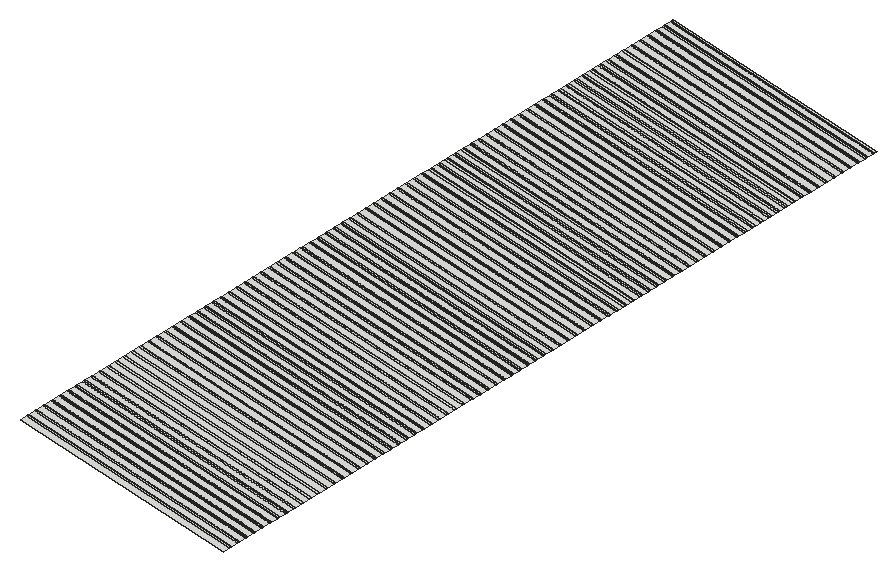
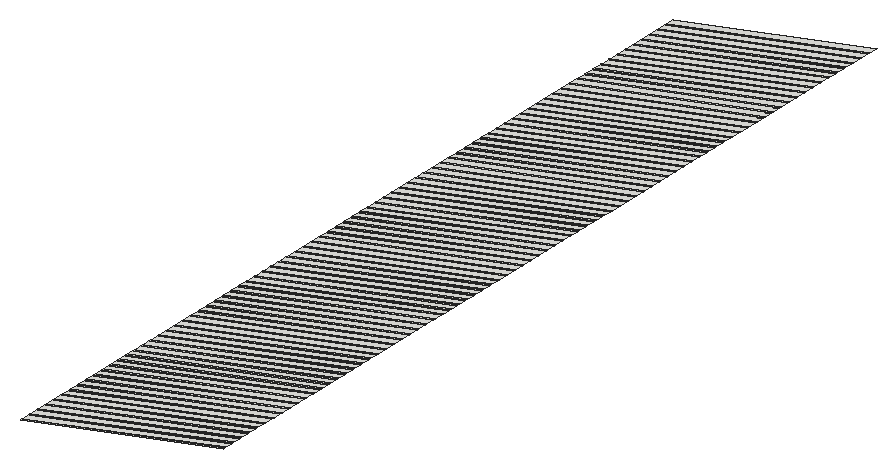
# SketchUp Ruby script. Lengths in inches.
U = 1.inch
M = Sketchup.active_model
def pt(a) = Geom::Point3d.new(a.map { |v| v * U })
def face(e, loops, mat)
  f = e.add_face(loops[0].map { |a| pt(a) })
  loops[1..].each { |l| e.add_face(l.map { |a| pt(a) }).erase! }
  f.material = f.back_material = mat if mat
  f
end
# faces: each face lists its corners as indices into pts; further lists are holes
def faces(e, pts, list, mat = nil) = list.each { |f| face(e, (f[0].is_a?(Array) ? f : [f]).map { |l| l.map { |i| pts[i] } }, mat) }
# xy, xz, yz: faces in a plane at the given z, y or x. An outline is a flat list of corners, or four numbers for a rectangle; further outlines are holes
def ring(l) = l.size == 4 ? [[l[0], l[1]], [l[2], l[1]], [l[2], l[3]], [l[0], l[3]]] : l.each_slice(2).to_a
def flat(e, list, mat, &to3) = list.each { |f| face(e, (f[0].is_a?(Array) ? f : [f]).map { |l| ring(l).map { |u, v| to3.(u, v) } }, mat) }
def xy(e, z, list, mat = nil) = flat(e, list, mat) { |x, y| [x, y, z] }
def xz(e, y, list, mat = nil) = flat(e, list, mat) { |x, z| [x, y, z] }
def yz(e, x, list, mat = nil) = flat(e, list, mat) { |y, z| [x, y, z] }
def lines(e, pts, list) = list.each { |a, b| e.add_line(pt(pts[a]), pt(pts[b])) }
# prism: a flat outline (further loops are holes) pulled along v
def prism(e, loops, v, mat = nil)
  f = face(e, loops, mat); d = Geom::Vector3d.new(v.map { |x| x * U })
  f.pushpull(f.normal.samedirection?(d) ? d.length : -d.length)
end
def box(e, o, s, mat = nil) = prism(e, [[o, [o[0] + s[0], o[1], o[2]], [o[0] + s[0], o[1] + s[1], o[2]], [o[0], o[1] + s[1], o[2]]]], [0, 0, s[2]], mat)
def at(x, y, z, deg = 0) = Geom::Transformation.translation(pt([x, y, z])) * Geom::Transformation.rotation(ORIGIN, Z_AXIS, deg.degrees)
def axes(o, x, y, z) = Geom::Transformation.new([*x, 0, *y, 0, *z, 0, *pt(o).to_a, 1])
def part(name) = M.definitions.add(name)
# library, detail: a bought-in or finely detailed component or shape, given as its bounding box
def library(name, o, s) = part(name).tap { |d| box(d.entities, o, s) }
def detail(e, o, s) = box(e.add_group.entities, o, s)
def put(e, d, t, mat = nil) = e.add_instance(d, t).tap { |i| i.material = mat if mat }
def group(e, t, mat = nil) = e.add_group.tap { |g| g.transformation = t; g.material = mat if mat }.entities
root = M.entities
p = [[2686.81,1547.47,214.83],[2686.81,1557.625,214.83],[2423.52,1558.75,274.66],[2423.52,1548.6,274.66],[2686.81,1559.59,214.83],[2423.52,1560.72,274.66],
  [2423.52,1561.61,274.66],[2686.81,1560.49,214.83],[2686.81,1570.62,214.83],[2423.52,1571.75,274.66],[2686.81,1572.59,214.83],[2423.52,1573.72,274.66],
  [2423.52,1574.625,274.66],[2686.81,1573.5,214.83],[2686.81,1583.62,214.83],[2423.52,1584.75,274.66],[2686.81,1585.59,214.83],[2423.52,1586.71,274.66],
  [2423.52,1587.64,274.66],[2686.81,1586.51,214.83],[2686.81,1596.62,214.83],[2423.52,1597.74,274.66],[2686.81,1598.59,214.83],[2423.52,1599.71,274.66],
  [2423.52,1600.65,274.66],[2686.81,1599.53,214.83],[2686.81,1609.62,214.83],[2423.52,1610.74,274.66],[2686.81,1611.58,214.83],[2423.52,1612.71,274.66],
  [2423.52,1613.67,274.66],[2686.81,1612.54,214.83],[2686.81,1622.61,214.83],[2423.52,1623.74,274.66],[2686.81,1624.58,214.83],[2423.52,1625.71,274.66],
  [2423.52,1626.68,274.66],[2686.81,1625.55,214.83],[2686.81,1635.61,214.83],[2423.52,1636.74,274.66],[2686.81,1637.58,214.83],[2423.52,1638.7,274.66],
  [2423.52,1639.69,274.66],[2686.81,1638.57,214.83],[2686.81,1648.61,214.83],[2423.52,1649.73,274.66],[2686.81,1650.58,214.83],[2423.52,1651.7,274.66],
  [2423.52,1652.71,274.66],[2686.81,1651.58,214.83],[2686.81,1661.61,214.83],[2423.52,1662.73,274.66],[2686.81,1663.57,214.83],[2423.52,1664.7,274.66],
  [2423.52,1665.72,274.66],[2686.81,1664.6,214.83],[2686.81,1674.6,214.83],[2423.52,1675.73,274.66],[2686.81,1676.57,214.83],[2423.52,1677.7,274.66],
  [2423.52,1678.73,274.66],[2686.81,1677.61,214.83],[2686.81,1687.6,214.83],[2423.52,1688.73,274.66],[2686.81,1689.57,214.83],[2423.52,1690.69,274.66],
  [2423.52,1691.75,274.66],[2686.81,1690.62,214.83],[2686.81,1700.6,214.83],[2423.52,1701.72,274.66],[2686.81,1702.57,214.83],[2423.52,1703.69,274.66],
  [2423.52,1704.76,274.66],[2686.81,1703.64,214.83],[2686.81,1713.6,214.83],[2423.52,1714.72,274.66],[2686.81,1715.5625,214.83],[2423.52,1716.6875,274.66],
  [2423.52,1717.77,274.66],[2686.81,1716.65,214.83],[2686.81,1726.59,214.83],[2423.52,1727.72,274.66],[2686.81,1728.5625,214.83],[2423.52,1729.6875,274.66],
  [2423.52,1730.79,274.66],[2686.81,1729.66,214.83],[2686.81,1739.59,214.83],[2423.52,1740.72,274.66],[2686.81,1741.56,214.83],[2423.52,1742.68,274.66],
  [2423.52,1743.8,274.66],[2686.81,1742.68,214.83],[2686.81,1752.59,214.83],[2423.52,1753.71,274.66],[2686.81,1754.56,214.83],[2423.52,1755.68,274.66],
  [2423.52,1756.8125,274.66],[2686.81,1755.6875,214.83],[2686.81,1765.59,214.83],[2423.52,1766.71,274.66],[2686.81,1767.55,214.83],[2423.52,1768.68,274.66],
  [2423.52,1769.83,274.66],[2686.81,1768.7,214.83],[2686.81,1778.58,214.83],[2423.52,1779.71,274.66],[2686.81,1780.55,214.83],[2423.52,1781.68,274.66],
  [2423.52,1782.84,274.66],[2686.81,1781.72,214.83],[2686.81,1791.58,214.83],[2423.52,1792.71,274.66],[2686.81,1793.55,214.83],[2423.52,1794.67,274.66],
  [2423.52,1795.85,274.66],[2686.81,1794.73,214.83],[2686.81,1804.58,214.83],[2423.52,1805.7,274.66],[2686.81,1806.55,214.83],[2423.52,1807.67,274.66],
  [2423.52,1808.87,274.66],[2686.81,1807.74,214.83],[2686.81,1817.58,214.83],[2423.52,1818.7,274.66],[2686.81,1819.54,214.83],[2423.52,1820.67,274.66],
  [2423.52,1821.88,274.66],[2686.81,1820.76,214.83],[2686.81,1830.57,214.83],[2423.52,1831.7,274.66],[2686.81,1832.54,214.83],[2423.52,1833.67,274.66],
  [2423.52,1834.89,274.66],[2686.81,1833.77,214.83],[2686.81,1843.57,214.83],[2423.52,1844.7,274.66],[2686.81,1845.54,214.83],[2423.52,1846.66,274.66],
  [2423.52,1847.91,274.66],[2686.81,1846.78,214.83],[2686.81,1856.57,214.83],[2423.52,1857.69,274.66],[2686.81,1858.54,214.83],[2423.52,1859.66,274.66],
  [2423.52,1860.92,274.66],[2686.81,1859.8,214.83],[2686.81,1869.57,214.83],[2423.52,1870.69,274.66],[2686.81,1871.53,214.83],[2423.52,1872.66,274.66],
  [2423.52,1873.94,274.66],[2686.81,1872.81,214.83],[2686.81,1882.5625,214.83],[2423.52,1883.6875,274.66],[2686.81,1884.53,214.83],[2423.52,1885.66,274.66],
  [2423.52,1886.95,274.66],[2686.81,1885.82,214.83],[2686.81,1895.5625,214.83],[2423.52,1896.6875,274.66],[2686.81,1897.53,214.83],[2423.52,1898.65,274.66],
  [2423.52,1899.96,274.66],[2686.81,1898.84,214.83],[2686.81,1908.56,214.83],[2423.52,1909.68,274.66],[2686.81,1910.53,214.83],[2423.52,1911.65,274.66],
  [2423.52,1912.98,274.66],[2686.81,1911.85,214.83],[2686.81,1921.56,214.83],[2423.52,1922.68,274.66],[2686.81,1923.52,214.83],[2423.52,1924.65,274.66],
  [2423.52,1925.99,274.66],[2686.81,1924.86,214.83],[2686.81,1934.55,214.83],[2423.52,1935.68,274.66],[2686.81,1936.52,214.83],[2423.52,1937.65,274.66],
  [2423.52,1939,274.66],[2686.81,1937.88,214.83],[2686.81,1947.55,214.83],[2423.52,1948.68,274.66],[2686.81,1949.52,214.83],[2423.52,1950.64,274.66],
  [2423.52,1952.02,274.66],[2686.81,1950.89,214.83],[2686.81,1960.55,214.83],[2423.52,1961.67,274.66],[2686.81,1962.52,214.83],[2423.52,1963.64,274.66],
  [2423.52,1965.03,274.66],[2686.81,1963.9,214.83],[2686.81,1973.55,214.83],[2423.52,1974.67,274.66],[2686.81,1975.51,214.83],[2423.52,1976.64,274.66],
  [2423.52,1978.04,274.66],[2686.81,1976.92,214.83],[2686.81,1986.54,214.83],[2423.52,1987.67,274.66],[2686.81,1988.51,214.83],[2423.52,1989.64,274.66],
  [2423.52,1991.06,274.66],[2686.81,1989.93,214.83],[2686.81,1999.54,214.83],[2423.52,2000.67,274.66],[2686.81,2001.51,214.83],[2423.52,2002.63,274.66],
  [2423.52,2004.07,274.66],[2686.81,2002.94,214.83],[2686.81,2012.54,214.83],[2423.52,2013.66,274.66],[2686.81,2014.51,214.83],[2423.52,2015.63,274.66],
  [2423.52,2017.08,274.66],[2686.81,2015.96,214.83],[2686.81,2025.54,214.83],[2423.52,2026.66,274.66],[2686.81,2027.5,214.83],[2423.52,2028.63,274.66],
  [2423.52,2030.1,274.66],[2686.81,2028.97,214.83],[2686.81,2038.53,214.83],[2423.52,2039.66,274.66],[2686.81,2040.5,214.83],[2423.52,2041.625,274.66],
  [2423.52,2043.11,274.66],[2686.81,2041.98,214.83],[2686.81,2051.53,214.83],[2423.52,2052.66,274.66],[2686.81,2053.5,214.83],[2423.52,2054.625,274.66],
  [2423.52,2056.125,274.66],[2686.81,2055,214.83],[2686.81,2064.53,214.83],[2423.52,2065.65,274.66],[2686.81,2066.5,214.83],[2423.52,2067.62,274.66],
  [2423.52,2069.14,274.66],[2686.81,2068.01,214.83],[2686.81,2077.53,214.83],[2423.52,2078.65,274.66],[2686.81,2079.49,214.83],[2423.52,2080.62,274.66],
  [2423.52,2082.15,274.66],[2686.81,2081.03,214.83],[2686.81,2090.52,214.83],[2423.52,2091.65,274.66],[2686.81,2092.49,214.83],[2423.52,2093.62,274.66],
  [2423.52,2095.16,274.66],[2686.81,2094.04,214.83],[2686.81,2103.52,214.83],[2423.52,2104.65,274.66],[2686.81,2105.49,214.83],[2423.52,2106.61,274.66],
  [2423.52,2108.18,274.66],[2686.81,2107.05,214.83],[2686.81,2116.52,214.83],[2423.52,2117.64,274.66],[2686.81,2118.49,214.83],[2423.52,2119.61,274.66],
  [2423.52,2121.19,274.66],[2686.81,2120.07,214.83],[2686.81,2129.52,214.83],[2423.52,2130.64,274.66],[2686.81,2131.48,214.83],[2423.52,2132.61,274.66],
  [2423.52,2134.2,274.66],[2686.81,2133.08,214.83],[2686.81,2142.51,214.83],[2423.52,2143.64,274.66],[2686.81,2144.48,214.83],[2423.52,2145.61,274.66],
  [2423.52,2147.22,274.66],[2686.81,2146.09,214.83],[2686.81,2155.51,214.83],[2423.52,2156.64,274.66],[2686.81,2157.48,214.83],[2423.52,2158.6,274.66],
  [2423.52,2160.23,274.66],[2686.81,2159.11,214.83],[2686.81,2168.51,214.83],[2423.52,2169.63,274.66],[2686.81,2170.48,214.83],[2423.52,2171.6,274.66],
  [2423.52,2173.24,274.66],[2686.81,2172.12,214.83],[2686.81,2181.51,214.83],[2423.52,2182.63,274.66],[2686.81,2183.47,214.83],[2423.52,2184.6,274.66],
  [2423.52,2186.26,274.66],[2686.81,2185.13,214.83],[2686.81,2194.5,214.83],[2423.52,2195.63,274.66],[2686.81,2196.47,214.83],[2423.52,2197.6,274.66],
  [2423.52,2199.27,274.66],[2686.81,2198.15,214.83],[2686.81,2207.5,214.83],[2423.52,2208.625,274.66],[2686.81,2209.47,214.83],[2423.52,2210.59,274.66],
  [2423.52,2212.28,274.66],[2686.81,2211.16,214.83],[2686.81,2220.5,214.83],[2423.52,2221.625,274.66],[2686.81,2222.47,214.83],[2423.52,2223.59,274.66],
  [2423.52,2225.3,274.66],[2686.81,2224.17,214.83],[2686.81,2233.5,214.83],[2423.52,2234.62,274.66],[2686.81,2235.46,214.83],[2423.52,2236.59,274.66],
  [2423.52,2238.3125,274.66],[2686.81,2237.1875,214.83],[2686.81,2246.49,214.83],[2423.52,2247.62,274.66],[2686.81,2248.46,214.83],[2423.52,2249.59,274.66],
  [2423.52,2251.32,274.66],[2686.81,2250.2,214.83],[2686.81,2259.49,214.83],[2423.52,2260.62,274.66],[2686.81,2261.46,214.83],[2423.52,2262.58,274.66],
  [2423.52,2264.34,274.66],[2686.81,2263.21,214.83],[2686.81,2272.49,214.83],[2423.52,2273.61,274.66],[2686.81,2274.46,214.83],[2423.52,2275.58,274.66],
  [2423.52,2277.35,274.66],[2686.81,2276.23,214.83],[2686.81,2285.49,214.83],[2423.52,2286.61,274.66],[2686.81,2287.45,214.83],[2423.52,2288.58,274.66],
  [2423.52,2290.37,274.66],[2686.81,2289.24,214.83],[2686.81,2298.48,214.83],[2423.52,2299.61,274.66],[2686.81,2300.45,214.83],[2423.52,2301.58,274.66],
  [2423.52,2303.38,274.66],[2686.81,2302.25,214.83],[2686.81,2311.48,214.83],[2423.52,2312.61,274.66],[2686.81,2313.45,214.83],[2423.52,2314.57,274.66],
  [2423.52,2316.39,274.66],[2686.81,2315.27,214.83],[2686.81,2324.48,214.83],[2423.52,2325.6,274.66],[2686.81,2326.45,214.83],[2423.52,2327.57,274.66],
  [2423.52,2329.41,274.66],[2686.81,2328.28,214.83],[2686.81,2337.48,214.83],[2423.52,2338.6,274.66],[2686.81,2339.44,214.83],[2423.52,2340.57,274.66],
  [2423.52,2342.42,274.66],[2686.81,2341.29,214.83],[2686.81,2350.47,214.83],[2423.52,2351.6,274.66],[2686.81,2352.44,214.83],[2423.52,2353.57,274.66],
  [2423.52,2355.43,274.66],[2686.81,2354.31,214.83],[2686.81,2363.47,214.83],[2423.52,2364.6,274.66],[2686.81,2365.44,214.83],[2423.52,2366.56,274.66],
  [2423.52,2368.45,274.66],[2686.81,2367.32,214.83],[2686.81,2376.47,214.83],[2423.52,2377.59,274.66],[2686.81,2378.4375,214.83],[2423.52,2379.5625,274.66],
  [2423.52,2381.46,274.66],[2686.81,2380.33,214.83],[2686.81,2389.47,214.83],[2423.52,2390.59,274.66],[2686.81,2391.43,214.83],[2423.52,2392.56,274.66],
  [2423.52,2394.47,274.66],[2686.81,2393.35,214.83],[2686.81,2402.46,214.83],[2423.52,2403.59,274.66],[2686.81,2404.43,214.83],[2423.52,2405.56,274.66],
  [2423.52,2407.49,274.66],[2686.81,2406.36,214.83],[2686.81,2415.46,214.83],[2423.52,2416.59,274.66],[2686.81,2417.43,214.83],[2423.52,2418.55,274.66],
  [2423.52,2420.5,274.66],[2686.81,2419.375,214.83],[2686.81,2428.46,214.83],[2423.52,2429.58,274.66],[2686.81,2430.43,214.83],[2423.52,2431.55,274.66],
  [2423.52,2433.51,274.66],[2686.81,2432.39,214.83],[2686.81,2441.46,214.83],[2423.52,2442.58,274.66],[2686.81,2443.42,214.83],[2423.52,2444.55,274.66],
  [2423.52,2446.53,274.66],[2686.81,2445.4,214.83],[2686.81,2454.45,214.83],[2423.52,2455.58,274.66],[2686.81,2456.42,214.83],[2423.52,2457.55,274.66],
  [2423.52,2459.54,274.66],[2686.81,2458.41,214.83],[2686.81,2467.45,214.83],[2423.52,2468.58,274.66],[2686.81,2469.42,214.83],[2423.52,2470.54,274.66],
  [2423.52,2472.55,274.66],[2686.81,2471.43,214.83],[2686.81,2480.45,214.83],[2423.52,2481.57,274.66],[2686.81,2482.42,214.83],[2423.52,2483.54,274.66],
  [2423.52,2485.57,274.66],[2686.81,2484.44,214.83],[2686.81,2493.45,214.83],[2423.52,2494.57,274.66],[2686.81,2495.41,214.83],[2423.52,2496.54,274.66],
  [2423.52,2498.58,274.66],[2686.81,2497.46,214.83],[2686.81,2506.44,214.83],[2423.52,2507.57,274.66],[2686.81,2508.41,214.83],[2423.52,2509.54,274.66],
  [2423.52,2511.59,274.66],[2686.81,2510.47,214.83],[2686.81,2519.44,214.83],[2423.52,2520.57,274.66],[2686.81,2521.41,214.83],[2423.52,2522.53,274.66],
  [2423.52,2524.61,274.66],[2686.81,2523.48,214.83],[2686.81,2532.4375,214.83],[2423.52,2533.5625,274.66],[2686.81,2534.41,214.83],[2423.52,2535.53,274.66],
  [2423.52,2537.62,274.66],[2686.81,2536.5,214.83],[2686.81,2545.4375,214.83],[2423.52,2546.5625,274.66],[2686.81,2547.4,214.83],[2423.52,2548.53,274.66],
  [2423.52,2550.63,274.66],[2686.81,2549.51,214.83],[2686.81,2558.43,214.83],[2423.52,2559.56,274.66],[2686.81,2560.4,214.83],[2423.52,2561.53,274.66],
  [2423.52,2563.65,274.66],[2686.81,2562.52,214.83],[2686.81,2571.43,214.83],[2423.52,2572.56,274.66],[2686.81,2573.4,214.83],[2423.52,2574.52,274.66],
  [2423.52,2576.66,274.66],[2686.81,2575.54,214.83],[2686.81,2584.43,214.83],[2423.52,2585.55,274.66],[2686.81,2586.4,214.83],[2423.52,2587.52,274.66],
  [2423.52,2589.67,274.66],[2686.81,2588.55,214.83],[2686.81,2597.43,214.83],[2423.52,2598.55,274.66],[2686.81,2599.39,214.83],[2423.52,2600.52,274.66],
  [2423.52,2602.6875,274.66],[2686.81,2601.5625,214.83]]
faces(root,p,[[0,1,2,3],[2,1,4,5],[6,5,4,7],[7,8,9,6],[9,8,10,11],[12,11,10,13],[13,14,15,12],[15,14,16,17],
  [18,17,16,19],[19,20,21,18],[21,20,22,23],[24,23,22,25],[25,26,27,24],[27,26,28,29],[30,29,28,31],[31,32,33,30],
  [33,32,34,35],[36,35,34,37],[37,38,39,36],[39,38,40,41],[42,41,40,43],[43,44,45,42],[45,44,46,47],[48,47,46,49],
  [49,50,51,48],[51,50,52,53],[54,53,52,55],[55,56,57,54],[57,56,58,59],[60,59,58,61],[61,62,63,60],[63,62,64,65],
  [66,65,64,67],[67,68,69,66],[69,68,70,71],[72,71,70,73],[73,74,75,72],[75,74,76,77],[78,77,76,79],[79,80,81,78],
  [81,80,82,83],[84,83,82,85],[85,86,87,84],[87,86,88,89],[90,89,88,91],[91,92,93,90],[93,92,94,95],[96,95,94,97],
  [97,98,99,96],[99,98,100,101],[102,101,100,103],[103,104,105,102],[105,104,106,107],[108,107,106,109],[109,110,111,108],[111,110,112,113],
  [114,113,112,115],[115,116,117,114],[117,116,118,119],[120,119,118,121],[121,122,123,120],[123,122,124,125],[126,125,124,127],[127,128,129,126],
  [129,128,130,131],[132,131,130,133],[133,134,135,132],[135,134,136,137],[138,137,136,139],[139,140,141,138],[141,140,142,143],[144,143,142,145],
  [145,146,147,144],[147,146,148,149],[150,149,148,151],[151,152,153,150],[153,152,154,155],[156,155,154,157],[157,158,159,156],[159,158,160,161],
  [162,161,160,163],[163,164,165,162],[165,164,166,167],[168,167,166,169],[169,170,171,168],[171,170,172,173],[174,173,172,175],[175,176,177,174],
  [177,176,178,179],[180,179,178,181],[181,182,183,180],[183,182,184,185],[186,185,184,187],[187,188,189,186],[189,188,190,191],[192,191,190,193],
  [193,194,195,192],[195,194,196,197],[198,197,196,199],[199,200,201,198],[201,200,202,203],[204,203,202,205],[205,206,207,204],[207,206,208,209],
  [210,209,208,211],[211,212,213,210],[213,212,214,215],[216,215,214,217],[217,218,219,216],[219,218,220,221],[222,221,220,223],[223,224,225,222],
  [225,224,226,227],[228,227,226,229],[229,230,231,228],[231,230,232,233],[234,233,232,235],[235,236,237,234],[237,236,238,239],[240,239,238,241],
  [241,242,243,240],[243,242,244,245],[246,245,244,247],[247,248,249,246],[249,248,250,251],[252,251,250,253],[253,254,255,252],[255,254,256,257],
  [258,257,256,259],[259,260,261,258],[261,260,262,263],[264,263,262,265],[265,266,267,264],[267,266,268,269],[270,269,268,271],[271,272,273,270],
  [273,272,274,275],[276,275,274,277],[277,278,279,276],[279,278,280,281],[282,281,280,283],[283,284,285,282],[285,284,286,287],[288,287,286,289],
  [289,290,291,288],[291,290,292,293],[294,293,292,295],[295,296,297,294],[297,296,298,299],[300,299,298,301],[301,302,303,300],[303,302,304,305],
  [306,305,304,307],[307,308,309,306],[309,308,310,311],[312,311,310,313],[313,314,315,312],[315,314,316,317],[318,317,316,319],[319,320,321,318],
  [321,320,322,323],[324,323,322,325],[325,326,327,324],[327,326,328,329],[330,329,328,331],[331,332,333,330],[333,332,334,335],[336,335,334,337],
  [337,338,339,336],[339,338,340,341],[342,341,340,343],[343,344,345,342],[345,344,346,347],[348,347,346,349],[349,350,351,348],[351,350,352,353],
  [354,353,352,355],[355,356,357,354],[357,356,358,359],[360,359,358,361],[361,362,363,360],[363,362,364,365],[366,365,364,367],[367,368,369,366],
  [369,368,370,371],[372,371,370,373],[373,374,375,372],[375,374,376,377],[378,377,376,379],[379,380,381,378],[381,380,382,383],[384,383,382,385],
  [385,386,387,384],[387,386,388,389],[390,389,388,391],[391,392,393,390],[393,392,394,395],[396,395,394,397],[397,398,399,396],[399,398,400,401],
  [402,401,400,403],[403,404,405,402],[405,404,406,407],[408,407,406,409],[409,410,411,408],[411,410,412,413],[414,413,412,415],[415,416,417,414],
  [417,416,418,419],[420,419,418,421],[421,422,423,420],[423,422,424,425],[426,425,424,427],[427,428,429,426],[429,428,430,431],[432,431,430,433],
  [433,434,435,432],[435,434,436,437],[438,437,436,439],[439,440,441,438],[441,440,442,443],[444,443,442,445],[445,446,447,444],[447,446,448,449],
  [450,449,448,451],[451,452,453,450],[453,452,454,455],[456,455,454,457],[457,458,459,456],[459,458,460,461],[462,461,460,463],[463,464,465,462],
  [465,464,466,467],[468,467,466,469],[469,470,471,468],[471,470,472,473],[474,473,472,475],[475,476,477,474],[477,476,478,479],[480,479,478,481],
  [481,482,483,480],[483,482,484,485],[486,485,484,487]])
